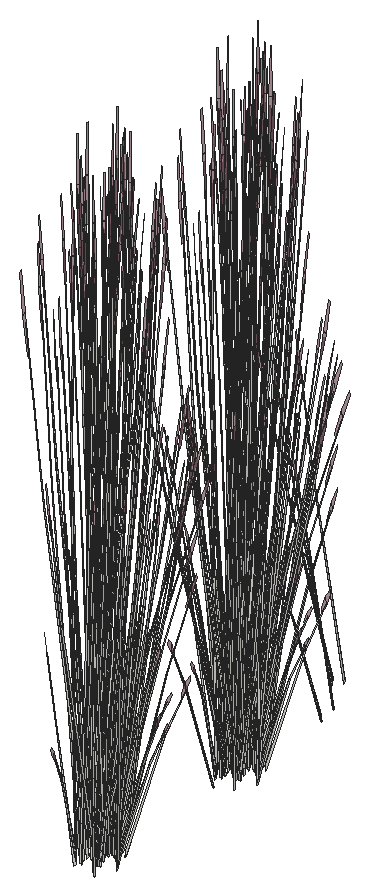
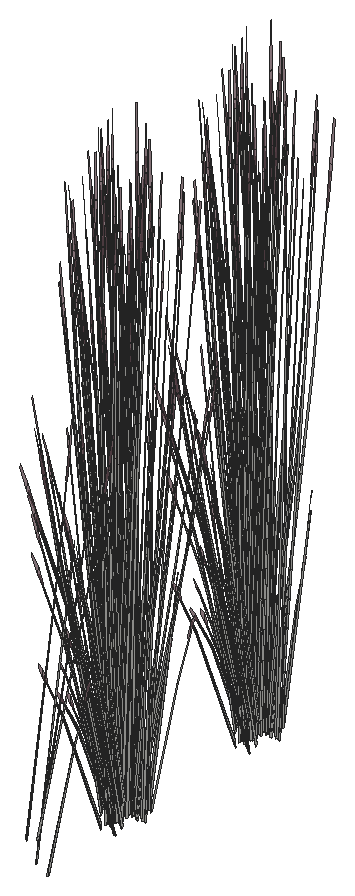
# SketchUp Ruby script. Lengths in inches.
U = 1.inch
M = Sketchup.active_model
def pt(a) = Geom::Point3d.new(a.map { |v| v * U })
def face(e, loops, mat)
  f = e.add_face(loops[0].map { |a| pt(a) })
  loops[1..].each { |l| e.add_face(l.map { |a| pt(a) }).erase! }
  f.material = f.back_material = mat if mat
  f
end
# faces: each face lists its corners as indices into pts; further lists are holes
def faces(e, pts, list, mat = nil) = list.each { |f| face(e, (f[0].is_a?(Array) ? f : [f]).map { |l| l.map { |i| pts[i] } }, mat) }
# xy, xz, yz: faces in a plane at the given z, y or x. An outline is a flat list of corners, or four numbers for a rectangle; further outlines are holes
def ring(l) = l.size == 4 ? [[l[0], l[1]], [l[2], l[1]], [l[2], l[3]], [l[0], l[3]]] : l.each_slice(2).to_a
def flat(e, list, mat, &to3) = list.each { |f| face(e, (f[0].is_a?(Array) ? f : [f]).map { |l| ring(l).map { |u, v| to3.(u, v) } }, mat) }
def xy(e, z, list, mat = nil) = flat(e, list, mat) { |x, y| [x, y, z] }
def xz(e, y, list, mat = nil) = flat(e, list, mat) { |x, z| [x, y, z] }
def yz(e, x, list, mat = nil) = flat(e, list, mat) { |y, z| [x, y, z] }
def lines(e, pts, list) = list.each { |a, b| e.add_line(pt(pts[a]), pt(pts[b])) }
# prism: a flat outline (further loops are holes) pulled along v
def prism(e, loops, v, mat = nil)
  f = face(e, loops, mat); d = Geom::Vector3d.new(v.map { |x| x * U })
  f.pushpull(f.normal.samedirection?(d) ? d.length : -d.length)
end
def box(e, o, s, mat = nil) = prism(e, [[o, [o[0] + s[0], o[1], o[2]], [o[0] + s[0], o[1] + s[1], o[2]], [o[0], o[1] + s[1], o[2]]]], [0, 0, s[2]], mat)
def at(x, y, z, deg = 0) = Geom::Transformation.translation(pt([x, y, z])) * Geom::Transformation.rotation(ORIGIN, Z_AXIS, deg.degrees)
def axes(o, x, y, z) = Geom::Transformation.new([*x, 0, *y, 0, *z, 0, *pt(o).to_a, 1])
def part(name) = M.definitions.add(name)
# library, detail: a bought-in or finely detailed component or shape, given as its bounding box
def library(name, o, s) = part(name).tap { |d| box(d.entities, o, s) }
def detail(e, o, s) = box(e.add_group.entities, o, s)
def put(e, d, t, mat = nil) = e.add_instance(d, t).tap { |i| i.material = mat if mat }
def group(e, t, mat = nil) = e.add_group.tap { |g| g.transformation = t; g.material = mat if mat }.entities
root = M.entities
M.materials.add("LightPink_Translucent").color = [144, 107, 117]
M.materials["LightPink_Translucent"].alpha = 0.75
c1 = part("blade")
p = [[2.15,0.21,22],[0,0.17,0],[0.09,0.45,0],[2.18,0.31,22],[2.29,0.31,22],[0.38,0.45,0],
  [2.48,0.24,33],[2.49,0.24,33],[2.48,0.22,33]]
faces(c1.entities,p,[[0,1,2,3],[4,5,2,3],[6,3,4,7],[8,0,3,6]])
c2 = part("seeds")
p = [[0.3,-0.1,1.38],[-0.01,-0.03,1.59],[-0.01,-0.03,0.03],[0.14,-0.07,-0.07],[0.29,-0.03,3],[0.15,0.01,3.11]]
faces(c2.entities,p,[[0,1,2,3],[1,0,4,5]],"LightPink_Translucent")
c3 = part("blade with seeds")
put(c3.entities,c1,at(0,0,0))
put(c3.entities,c2,axes([2.4,0.25,30.99],[1.5799,-0.05474,1.17369],[-0.12525,1.92788,0.29478],[-0.07173,-0.02425,1.56792]))
put(root,c3,axes([402.35,721.51,2.77],[0.04528,0.27194,1.1486],[-0.25117,-0.15062,0.84392],[0.02703,-0.13924,0.25299]))
put(root,c3,axes([402.89,722.82,4.68],[-0.25266,-0.31335,-0.51099],[0.2669,-0.27442,-0.3958],[0.03844,-0.15921,0.97773]))
put(root,c3,axes([403.13,722.7,4.53],[0.23881,-0.24554,-0.35414],[0.22606,0.28036,0.4572],[0.0344,-0.14245,0.87481]))
put(root,c3,axes([401.49,724.01,2.1],[-0.14494,-0.47823,-0.69835],[0.41752,-0.17223,-0.18329],[-0.01602,-0.16194,1.54149]))
put(root,c3,axes([403.43,722.55,1.49],[-0.05283,-0.03674,1.76342],[-0.13569,-0.41045,-0.26939],[0.09154,-0.11138,0.30037]))
put(root,c3,axes([403.42,723.71,4.98],[0.18436,-0.36797,-0.71045],[0.32306,0.26151,0.08574],[0.11008,-0.13332,1.00501]))
put(root,c3,axes([401.43,722.64,2.375],[-0.22066,-0.46731,0],[0.36918,-0.26061,-0.51607],[0.08408,-0.05936,1.63711]))
put(root,c3,axes([403.41,723.54,4.68],[-0.09067,-0.42583,-0.51099],[0.34336,-0.07449,-0.3958],[0.0984,-0.11438,0.97773]))
put(root,c3,axes([401.92,722.07,2.13],[-0.2439,0.26754,-0.03893],[-0.22348,-0.29302,-0.17649],[-0.01573,-0.08303,0.58215]))
put(root,c3,axes([400.63,723.95,2.02],[0,-0.46636,-0.49651],[0.39487,0,0],[0,-0.10622,1.57504]))
put(root,c3,axes([401.73,722.57,2.02],[0.33032,-0.23318,-0.49651],[0.19744,0.41812,0],[0.07523,-0.05311,1.57504]))
put(root,c3,axes([403.69,723.37,2.59],[-0.12609,-0.01381,1.43002],[-0.12917,-0.37055,-0.30754],[0.1549,-0.10482,0.61141]))
put(root,c3,axes([402.12,723.52,2.06],[0.23773,-0.35053,-0.62353],[0.29532,0.31785,-0.16365],[0.09526,-0.08744,1.37633]))
put(root,c3,axes([403.84,722.69,2.77],[-0.11756,0.2374,1.1486],[-0.10105,-0.31895,0.84392],[0.09709,-0.07992,0.25299]))
put(root,c3,axes([403.67,723.58,4.53],[0.30722,-0.06665,-0.35414],[0.08112,0.381,0.4572],[0.08804,-0.10234,0.87481]))
put(root,c3,axes([401.71,724.14,2.21],[0.17124,-0.42022,-0.44739],[0.35581,0.20224,0.21531],[0,-0.09687,1.43643]))
put(root,c3,axes([401.86,723.93,2.67],[-0.04113,-0.53214,-0.29095],[0.42835,-0.03218,-0.50002],[0.07543,-0.07088,1.59708]))
put(root,c3,axes([400.8,723.96,2.03],[0.24637,-0.29097,-0.30978],[0.24637,0.29097,0.30978],[0,-0.09372,1.38974]))
put(root,c3,axes([401.67,724.49,2.67],[-0.39748,-0.22252,-0.29095],[0.19139,-0.46966,-0.50002],[-0.01249,-0.11531,1.59708]))
put(root,c3,axes([401.81,722.75,2.03],[0.32928,0.11539,-0.30978],[-0.08291,0.40636,0.30978],[0.06638,-0.04686,1.38974]))
put(root,c3,axes([401.92,724.34,2.43],[0.39767,0.22603,0.24065],[-0.19139,0.46966,0.50002],[0,-0.10827,1.60543]))
put(root,c3,axes([401.79,724.03,2.72],[-0.38326,0.02879,0.44739],[-0.03466,-0.47788,-0.21531],[0.06861,-0.04843,1.43643]))
put(root,c3,axes([400.8,724.38,2.48],[0,0.46636,0.49651],[-0.39487,0,0],[0,-0.10622,1.57504]))
put(root,c3,axes([403.57,724.48,4.68],[0.09562,-0.42421,-0.51099],[0.32782,0.1454,-0.3958],[0.13199,-0.0389,0.97773]))
put(root,c3,axes([403.06,722.76,2.375],[0.22066,-0.46731,0],[0.36918,0.26061,-0.51607],[0.08408,0.05936,1.63711]))
put(root,c3,axes([401.78,724.2,2.36],[0.15345,0.52148,0.45755],[-0.43845,0.18134,0.17955],[0.00536,-0.09582,1.58856]))
put(root,c3,axes([403.92,724.6,1.98],[-0.22732,0.05597,1.41583],[-0.03618,-0.44548,0.08104],[0.15921,-0.06743,0.80566]))
put(root,c3,axes([404.34,724.21,2.26],[-0.21881,-0.29821,-0.06488],[0.23965,-0.27324,-0.29416],[0.0679,-0.01924,0.97024]))
put(root,c3,axes([401.7,724.61,2.72],[-0.17124,0.42022,0.44739],[-0.35581,-0.20224,-0.21531],[0,-0.09687,1.43643]))
put(root,c3,axes([402.33,724.25,2.21],[0,-0.53961,0],[0.44133,0,0],[0,0,1.79456]))
put(root,c3,axes([402.87,723,2.48],[-0.33032,-0.23318,0.49651],[0.19744,-0.41812,0],[0.07523,0.05311,1.57504]))
put(root,c3,axes([403.51,724.64,4.98],[0.31014,-0.20596,-0.71045],[0.17284,0.42397,0.08574],[0.14985,-0.04816,1.00501]))
put(root,c3,axes([402.12,723.91,2.36],[-0.29264,0.42323,0.45755],[-0.34767,-0.3736,0.17955],[0.07055,-0.04224,1.58856]))
put(root,c3,axes([402.44,724.66,2.3],[-0.32829,-0.4014,-0.06131],[0.32849,-0.40164,0],[-0.01146,-0.01402,1.75571]))
put(root,c3,axes([401.61,723.21,2.47],[-0.10196,0.46348,0.17642],[-0.3731,-0.13116,0.35086],[0.06445,-0.00226,1.60407]))
put(root,c3,axes([401.46,723.58,1.59],[-0.3474,0.18671,1.28929],[-0.11057,-0.53572,0.50096],[0.21332,0.00891,1.46642]))
put(root,c3,axes([402.39,723.72,2.62],[0.06809,-0.4162,0.1448],[0.33266,0.07225,-0.41347],[0.06054,0.04274,1.26744]))
put(root,c3,axes([401.82,724.71,2.36],[0.44609,0.09826,0.45755],[-0.09078,0.55493,0.17955],[-0.06519,-0.05359,1.58856]))
put(root,c3,axes([404.17,724.3125,1.49],[-0.01845,-0.0708,1.76342],[0.12793,-0.41416,-0.26939],[0.12905,-0.00596,0.30037]))
put(root,c3,axes([402.25,723.83,2.72],[-0.21202,-0.39143,0.44739],[0.32115,-0.27564,-0.21531],[0.06861,0.04843,1.43643]))
put(root,c3,axes([401.58,725.6,2.47],[0.37926,-0.12378,0.17642],[0.09365,0.46065,0.35086],[-0.03382,-0.06712,1.60407]))
put(root,c3,axes([402.36,723.86,2.67],[0.35635,-0.30962,-0.29095],[0.23697,0.43749,-0.50002],[0.08792,0.04443,1.59708]))
put(root,c3,axes([403.78,724.68,4.53],[0.29332,0.1301,-0.35414],[-0.08555,0.37955,0.4572],[0.11809,-0.0348,0.87481]))
put(root,c3,axes([403.26,723.04,2.02],[0.33032,0.23318,-0.49651],[-0.19744,0.41812,0],[0.07523,0.05311,1.57504]))
put(root,c3,axes([402.63,724.37,2.21],[0.39487,0,0],[0,0.48281,0],[0,0,1.78407]))
put(root,c3,axes([402.74,723.23,2.47],[-0.37926,0.12378,0.17642],[-0.09365,-0.46065,0.35086],[0.03382,0.06712,1.60407]))
put(root,c3,axes([402.98,724.21,3.875],[-0.14639,0.01056,1.71376],[0.09712,-0.45778,0.13857],[0.20862,0.02831,0.73262]))
put(root,c3,axes([403.17,723.21,2.03],[0.08291,0.40636,-0.30978],[-0.32928,0.11539,0.30978],[0.06638,0.04686,1.38974]))
put(root,c3,axes([402.5,724.12,2.38],[-0.44609,-0.09826,0.49198],[0.09078,-0.55493,0.19306],[0.06519,0.05359,1.70813]))
put(root,c3,axes([402.15,725.49,2.2],[-0.11516,-0.40207,0],[0.32884,-0.1408,0],[0,0,1.54371]))
put(root,c3,axes([402.58,725.43,2.18],[0.37054,-0.15823,-0.19198],[0.1302,0.45581,0.00008],[0.0409,-0.01749,1.73897]))
put(root,c3,axes([402.71,725.625,2.47],[0.10196,-0.46348,0.17642],[0.3731,0.13116,0.35086],[-0.06445,0.00226,1.60407]))
put(root,c3,axes([402.62,724.57,2.21],[0.24637,0.30123,0],[-0.24637,0.30123,0],[0,0,1.69266]))
put(root,c3,axes([403.29,724.44,2.47],[-0.2773,-0.3397,0.17642],[0.27945,-0.32949,0.35086],[-0.03063,0.06937,1.60407]))
put(root,c3,axes([402.78,723.93,2.06],[0.36714,0.07646,-0.62353],[-0.07747,0.47163,-0.16365],[0.10956,0.05715,1.37633]))
put(root,c3,axes([404.4,724.75,2.77],[-0.21807,0.07699,1.1486],[0.10265,-0.31819,0.84392],[0.11568,0.02177,0.25299]))
put(root,c3,axes([402.07,725.67,2.2],[-0.35581,-0.20937,0],[0.17124,-0.43505,0],[0,0,1.62707]))
put(root,c3,axes([402.62,724.22,2.72],[0.17124,-0.42022,0.44739],[0.35581,0.20224,-0.21531],[0,0.09687,1.43643]))
put(root,c3,axes([402.55,724.46,2.29],[0,0.53934,-0.05637],[-0.44133,0,0],[0,0.01695,1.79368]))
put(root,c3,axes([402.58,724.08,2.21],[0.21202,0.39143,-0.44739],[-0.32115,0.27564,0.21531],[0.06861,0.04843,1.43643]))
put(root,c3,axes([404.02,725.73,3.93],[-0.06755,-0.39203,-0.03492],[0.31928,-0.09013,-0.15832],[0.06667,0.02485,0.52218]))
put(root,c3,axes([403.52,724.46,2.48],[0,-0.46636,0.49651],[0.39487,0,0],[0,0.10622,1.57504]))
put(root,c3,axes([402.53,724.8,2.72],[0.38326,-0.02879,0.44739],[0.03466,0.47788,-0.21531],[-0.06861,0.04843,1.43643]))
put(root,c3,axes([402.77,724.32,2.62],[0.32884,-0.136,0.1448],[0.11516,0.38837,-0.41347],[0,0.08547,1.26744]))
put(root,c3,axes([403.99,725.26,2.59],[-0.085,-0.1147,1.43002],[0.1106,-0.37943,-0.30754],[0.17198,0.0514,0.61141]))
put(root,c3,axes([402.47,725.68,2.2],[0.35581,0.20937,0],[-0.17124,0.43505,0],[0,0,1.74954]))
put(root,c3,axes([402.61,726.14,2.19],[-0.21791,-0.46895,-0.05142],[0.36918,-0.26061,0.51607],[-0.09097,0.04465,1.6363]))
put(root,c3,axes([402.53,725.01,2.62],[0.26075,0.2802,0.1448],[-0.2175,0.31612,-0.41347],[-0.06054,0.04274,1.26744]))
put(root,c3,axes([403.21,725.49,4.98],[0.35281,0.01123,-0.71045],[-0.0237,0.47284,0.08574],[0.14947,0.0499,1.00501]))
put(root,c3,axes([402.8125,725.875,2.48],[0.33032,-0.23318,0.49651],[0.19744,0.41812,0],[-0.07523,0.05311,1.57504]))
put(root,c3,axes([402.34,725.51,2.29],[0.15345,0.53576,-0.06012],[-0.43845,0.18773,0],[0.00536,0.01871,1.72173]))
put(root,c3,axes([402.51,726.08,2.03],[-0.32928,-0.11539,-0.30978],[0.08291,-0.40636,0.30978],[-0.06638,0.04686,1.38974]))
put(root,c3,axes([403.78,724.53,2.375],[0.44133,0,0],[0,0.52122,-0.51607],[0,0.11871,1.63711]))
put(root,c3,axes([403.61,724.8,2.2],[-0.44111,-0.00373,-0.04976],[0,-0.52122,0.49943],[-0.01386,0.11865,1.58352]))
put(root,c3,axes([402.65,724.35,2.67],[0.39748,0.22252,-0.29095],[-0.19139,0.46966,-0.50002],[0.01249,0.11531,1.59708]))
put(root,c3,axes([403.42,725.6875,4.53],[0.20082,0.29199,-0.35414],[-0.2293,0.2764,0.4572],[0.1165,0.04206,0.87481]))
put(root,c3,axes([403.52,724.88,2.03],[-0.24637,0.29097,-0.30978],[-0.24637,-0.29097,0.30978],[0,0.09372,1.38974]))
put(root,c3,axes([402.46,724.91,2.67],[0.04113,0.53214,-0.29095],[-0.42835,0.03218,-0.50002],[-0.07543,0.07088,1.59708]))
put(root,c3,axes([402.61,724.7,2.21],[-0.17124,0.42022,-0.44739],[-0.35581,-0.20224,0.21531],[0,0.09687,1.43643]))
put(root,c3,axes([402.62,725.9,2.33],[0.44186,0.15158,0.30756],[-0.11054,0.54181,-0.36492],[-0.07313,0.06781,1.64885]))
put(root,c3,axes([402.59,726.27,2.02],[-0.33032,0.23318,-0.49651],[-0.19744,-0.41812,0],[-0.07523,0.05311,1.57504]))
put(root,c3,axes([403.6875,724.89,2.02],[0,0.46636,-0.49651],[-0.39487,0,0],[0,0.10622,1.57504]))
put(root,c3,axes([402.7,724.94,3.875],[-0.1311,-0.08035,1.71376],[0.27131,-0.33708,0.13857],[0.16909,0.15206,0.73262]))
put(root,c3,axes([403.18,725.86,2.77],[-0.19872,-0.13409,1.1486],[0.2566,-0.13625,0.84392],[0.06921,0.11541,0.25299]))
put(root,c3,axes([402.89,726.2,2.375],[0.22066,0.46731,0],[-0.36918,0.26061,-0.51607],[-0.08408,0.05936,1.63711]))
put(root,c3,axes([403.24,726.35,1.49],[0.02571,-0.06733,1.76342],[0.32373,-0.19829,-0.26939],[0.09815,0.10263,0.30037]))
put(root,c3,axes([402.7,724.35,2.84],[-0.00964,-0.43909,1.41272],[0.43635,0.11382,0.59816],[-0.1032,0.24027,1.3335]))
put(root,c3,axes([402.8125,724.82,2.09],[0.12941,0.42699,-0.69212],[-0.37279,0.15378,-0.18165],[0.0143,0.14459,1.52773]))
put(root,c3,axes([402.74,726.04,4.68],[0.34827,-0.11086,-0.51099],[0.06092,0.41983,-0.3958],[0.09354,0.12031,0.97773]))
put(root,c3,axes([403.22,726.47,2.67],[-0.22633,-0.01463,1.0506],[0.14947,-0.31064,0.58006],[0.08941,0.11036,0.8241]))
put(root,c3,axes([402.48,725.71,2.59],[0.00623,-0.15459,1.43002],[0.29764,-0.17268,-0.30754],[0.09188,0.18503,0.61141]))
put(root,c3,axes([401.73,726.34,1.49],[0.05712,-0.02538,1.76342],[0.34359,0.13968,-0.26939],[0.01005,0.15742,0.30037]))
put(root,c3,axes([401.21,725.93,5],[0.25266,0.31335,-0.5672],[-0.2669,0.27442,-0.43934],[-0.03844,0.15921,1.08528]))
put(root,c3,axes([400.9375,726.4,2.82],[0.32063,-0.08258,0.06507],[0.07371,0.33271,-0.86304],[-0.02033,0.16842,0.7736]))
put(root,c3,axes([401.96,726.24,4.68],[0.34695,0.11691,-0.51099],[-0.11892,0.40083,-0.3958],[0.03181,0.16138,0.97773]))
put(root,c3,axes([402.16,725.41,3.875],[-0.08068,-0.14973,1.71376],[0.3728,-0.12606,0.13857],[0.08426,0.23506,0.73262]))
put(root,c3,axes([401.8,726.48,4.53],[-0.1064,0.35863,-0.35414],[-0.31043,-0.1046,0.4572],[0.02846,0.14439,0.87481]))
put(root,c3,axes([401.5,725.48,3.875],[-0.00864,-0.17899,1.71376],[0.37441,0.11874,0.13857],[-0.02316,0.25508,0.73262]))
put(root,c3,axes([401.84,726.16,4.98],[0.16845,0.3792,-0.71045],[-0.34676,0.21133,0.08574],[0.03939,0.18322,1.00501]))
put(root,c3,axes([402.72,739.41,2.59],[-0.10032,0.0944,1.43002],[-0.30046,-0.16522,-0.30754],[0.05569,-0.20547,0.61141]))
put(root,c3,axes([402.27,739.73,4.98],[-0.16845,-0.3792,-0.71045],[0.34676,-0.21133,0.08574],[-0.03939,-0.18322,1.00501]))
put(root,c3,axes([401.98,738.89,1.49],[-0.0592,0.0168,1.76342],[-0.32738,-0.18913,-0.26939],[0.00549,-0.15776,0.30037]))
put(root,c3,axes([402.97,740.11,4.98],[0.00918,-0.43138,-0.71045],[0.38672,0.02897,0.08574],[0.04081,-0.18275,1.00501]))
put(root,c3,axes([402.3,739.41,4.53],[0.1064,-0.35863,-0.35414],[0.31043,0.1046,0.4572],[-0.02846,-0.14439,0.87481]))
put(root,c3,axes([402.53,739.89,3.875],[-0.06572,0.16029,1.71376],[-0.27569,-0.33172,0.13857],[0.12437,-0.20675,0.73262]))
put(root,c3,axes([402.14,739.66,4.68],[-0.34695,-0.11691,-0.51099],[0.11892,-0.40083,-0.3958],[-0.03181,-0.16138,0.97773]))
put(root,c3,axes([402.35,738.65,2.77],[0.04528,0.27194,1.1486],[-0.25117,-0.15062,0.84392],[0.02703,-0.13924,0.25299]))
put(root,c3,axes([402.89,739.96,4.68],[-0.25266,-0.31335,-0.51099],[0.2669,-0.27442,-0.3958],[0.03844,-0.15921,0.97773]))
put(root,c3,axes([403.13,739.85,4.53],[0.23881,-0.24554,-0.35414],[0.22606,0.28036,0.4572],[0.0344,-0.14245,0.87481]))
put(root,c3,axes([401.49,741.16,2.1],[-0.14494,-0.47823,-0.69835],[0.41752,-0.17223,-0.18329],[-0.01602,-0.16194,1.54149]))
put(root,c3,axes([403.43,739.7,1.49],[-0.05283,-0.03674,1.76342],[-0.13569,-0.41045,-0.26939],[0.09154,-0.11138,0.30037]))
put(root,c3,axes([403.42,740.86,4.98],[0.18436,-0.36797,-0.71045],[0.32306,0.26151,0.08574],[0.11008,-0.13332,1.00501]))
put(root,c3,axes([401.43,739.78,2.375],[-0.22066,-0.46731,0],[0.36918,-0.26061,-0.51607],[0.08408,-0.05936,1.63711]))
put(root,c3,axes([403.41,740.68,4.68],[-0.09067,-0.42583,-0.51099],[0.34336,-0.07449,-0.3958],[0.0984,-0.11438,0.97773]))
put(root,c3,axes([401.92,739.22,2.13],[-0.2439,0.26754,-0.03893],[-0.22348,-0.29302,-0.17649],[-0.01573,-0.08303,0.58215]))
put(root,c3,axes([400.63,741.09,2.02],[0,-0.46636,-0.49651],[0.39487,0,0],[0,-0.10622,1.57504]))
put(root,c3,axes([401.73,739.71,2.02],[0.33032,-0.23318,-0.49651],[0.19744,0.41812,0],[0.07523,-0.05311,1.57504]))
put(root,c3,axes([403.69,740.52,2.59],[-0.12609,-0.01381,1.43002],[-0.12917,-0.37055,-0.30754],[0.1549,-0.10482,0.61141]))
put(root,c3,axes([402.12,740.67,2.06],[0.23773,-0.35053,-0.62353],[0.29532,0.31785,-0.16365],[0.09526,-0.08744,1.37633]))
put(root,c3,axes([403.84,739.84,2.77],[-0.11756,0.2374,1.1486],[-0.10105,-0.31895,0.84392],[0.09709,-0.07992,0.25299]))
put(root,c3,axes([403.67,740.73,4.53],[0.30722,-0.06665,-0.35414],[0.08112,0.381,0.4572],[0.08804,-0.10234,0.87481]))
put(root,c3,axes([401.71,741.28,2.21],[0.17124,-0.42022,-0.44739],[0.35581,0.20224,0.21531],[0,-0.09687,1.43643]))
put(root,c3,axes([401.86,741.07,2.67],[-0.04113,-0.53214,-0.29095],[0.42835,-0.03218,-0.50002],[0.07543,-0.07088,1.59708]))
put(root,c3,axes([400.8,741.1,2.03],[0.24637,-0.29097,-0.30978],[0.24637,0.29097,0.30978],[0,-0.09372,1.38974]))
put(root,c3,axes([401.67,741.63,2.67],[-0.39748,-0.22252,-0.29095],[0.19139,-0.46966,-0.50002],[-0.01249,-0.11531,1.59708]))
put(root,c3,axes([401.81,739.9,2.03],[0.32928,0.11539,-0.30978],[-0.08291,0.40636,0.30978],[0.06638,-0.04686,1.38974]))
put(root,c3,axes([401.92,741.49,2.43],[0.39767,0.22603,0.24065],[-0.19139,0.46966,0.50002],[0,-0.10827,1.60543]))
put(root,c3,axes([401.79,741.18,2.72],[-0.38326,0.02879,0.44739],[-0.03466,-0.47788,-0.21531],[0.06861,-0.04843,1.43643]))
put(root,c3,axes([400.8,741.53,2.48],[0,0.46636,0.49651],[-0.39487,0,0],[0,-0.10622,1.57504]))
put(root,c3,axes([403.57,741.63,4.68],[0.09562,-0.42421,-0.51099],[0.32782,0.1454,-0.3958],[0.13199,-0.0389,0.97773]))
put(root,c3,axes([403.06,739.9,2.375],[0.22066,-0.46731,0],[0.36918,0.26061,-0.51607],[0.08408,0.05936,1.63711]))
put(root,c3,axes([401.78,741.35,2.36],[0.15345,0.52148,0.45755],[-0.43845,0.18134,0.17955],[0.00536,-0.09582,1.58856]))
put(root,c3,axes([403.92,741.75,1.98],[-0.22732,0.05597,1.41583],[-0.03618,-0.44548,0.08104],[0.15921,-0.06743,0.80566]))
put(root,c3,axes([404.34,741.35,2.26],[-0.21881,-0.29821,-0.06488],[0.23965,-0.27324,-0.29416],[0.0679,-0.01924,0.97024]))
put(root,c3,axes([401.7,741.76,2.72],[-0.17124,0.42022,0.44739],[-0.35581,-0.20224,-0.21531],[0,-0.09687,1.43643]))
put(root,c3,axes([402.33,741.39,2.21],[0,-0.53961,0],[0.44133,0,0],[0,0,1.79456]))
put(root,c3,axes([402.87,740.15,2.48],[-0.33032,-0.23318,0.49651],[0.19744,-0.41812,0],[0.07523,0.05311,1.57504]))
put(root,c3,axes([403.51,741.78,4.98],[0.31014,-0.20596,-0.71045],[0.17284,0.42397,0.08574],[0.14985,-0.04816,1.00501]))
put(root,c3,axes([402.12,741.05,2.36],[-0.29264,0.42323,0.45755],[-0.34767,-0.3736,0.17955],[0.07055,-0.04224,1.58856]))
put(root,c3,axes([402.44,741.8125,2.3],[-0.32829,-0.4014,-0.06131],[0.32849,-0.40164,0],[-0.01146,-0.01402,1.75571]))
put(root,c3,axes([401.61,740.36,2.47],[-0.10196,0.46348,0.17642],[-0.3731,-0.13116,0.35086],[0.06445,-0.00226,1.60407]))
put(root,c3,axes([401.46,740.73,1.59],[-0.3474,0.18671,1.28929],[-0.11057,-0.53572,0.50096],[0.21332,0.00891,1.46642]))
put(root,c3,axes([402.39,740.87,2.62],[0.06809,-0.4162,0.1448],[0.33266,0.07225,-0.41347],[0.06054,0.04274,1.26744]))
put(root,c3,axes([401.82,741.86,2.36],[0.44609,0.09826,0.45755],[-0.09078,0.55493,0.17955],[-0.06519,-0.05359,1.58856]))
put(root,c3,axes([404.17,741.46,1.49],[-0.01845,-0.0708,1.76342],[0.12793,-0.41416,-0.26939],[0.12905,-0.00596,0.30037]))
put(root,c3,axes([402.25,740.98,2.72],[-0.21202,-0.39143,0.44739],[0.32115,-0.27564,-0.21531],[0.06861,0.04843,1.43643]))
put(root,c3,axes([401.58,742.75,2.47],[0.37926,-0.12378,0.17642],[0.09365,0.46065,0.35086],[-0.03382,-0.06712,1.60407]))
put(root,c3,axes([402.36,741.01,2.67],[0.35635,-0.30962,-0.29095],[0.23697,0.43749,-0.50002],[0.08792,0.04443,1.59708]))
put(root,c3,axes([403.78,741.82,4.53],[0.29332,0.1301,-0.35414],[-0.08555,0.37955,0.4572],[0.11809,-0.0348,0.87481]))
put(root,c3,axes([403.26,740.18,2.02],[0.33032,0.23318,-0.49651],[-0.19744,0.41812,0],[0.07523,0.05311,1.57504]))
put(root,c3,axes([402.63,741.51,2.21],[0.39487,0,0],[0,0.48281,0],[0,0,1.78407]))
put(root,c3,axes([402.74,740.38,2.47],[-0.37926,0.12378,0.17642],[-0.09365,-0.46065,0.35086],[0.03382,0.06712,1.60407]))
put(root,c3,axes([402.98,741.35,3.875],[-0.14639,0.01056,1.71376],[0.09712,-0.45778,0.13857],[0.20862,0.02831,0.73262]))
put(root,c3,axes([403.17,740.36,2.03],[0.08291,0.40636,-0.30978],[-0.32928,0.11539,0.30978],[0.06638,0.04686,1.38974]))
put(root,c3,axes([402.5,741.27,2.38],[-0.44609,-0.09826,0.49198],[0.09078,-0.55493,0.19306],[0.06519,0.05359,1.70813]))
put(root,c3,axes([402.15,742.64,2.2],[-0.11516,-0.40207,0],[0.32884,-0.1408,0],[0,0,1.54371]))
put(root,c3,axes([402.58,742.58,2.18],[0.37054,-0.15823,-0.19198],[0.1302,0.45581,0.00008],[0.0409,-0.01749,1.73897]))
put(root,c3,axes([402.71,742.77,2.47],[0.10196,-0.46348,0.17642],[0.3731,0.13116,0.35086],[-0.06445,0.00226,1.60407]))
put(root,c3,axes([402.62,741.72,2.21],[0.24637,0.30123,0],[-0.24637,0.30123,0],[0,0,1.69266]))
put(root,c3,axes([403.29,741.59,2.47],[-0.2773,-0.3397,0.17642],[0.27945,-0.32949,0.35086],[-0.03063,0.06937,1.60407]))
put(root,c3,axes([402.78,741.08,2.06],[0.36714,0.07646,-0.62353],[-0.07747,0.47163,-0.16365],[0.10956,0.05715,1.37633]))
put(root,c3,axes([404.4,741.9,2.77],[-0.21807,0.07699,1.1486],[0.10265,-0.31819,0.84392],[0.11568,0.02177,0.25299]))
put(root,c3,axes([402.07,742.82,2.2],[-0.35581,-0.20937,0],[0.17124,-0.43505,0],[0,0,1.62707]))
put(root,c3,axes([402.62,741.37,2.72],[0.17124,-0.42022,0.44739],[0.35581,0.20224,-0.21531],[0,0.09687,1.43643]))
put(root,c3,axes([402.55,741.61,2.29],[0,0.53934,-0.05637],[-0.44133,0,0],[0,0.01695,1.79368]))
put(root,c3,axes([402.58,741.23,2.21],[0.21202,0.39143,-0.44739],[-0.32115,0.27564,0.21531],[0.06861,0.04843,1.43643]))
put(root,c3,axes([404.02,742.88,3.93],[-0.06755,-0.39203,-0.03492],[0.31928,-0.09013,-0.15832],[0.06667,0.02485,0.52218]))
put(root,c3,axes([403.52,741.6,2.48],[0,-0.46636,0.49651],[0.39487,0,0],[0,0.10622,1.57504]))
put(root,c3,axes([402.53,741.95,2.72],[0.38326,-0.02879,0.44739],[0.03466,0.47788,-0.21531],[-0.06861,0.04843,1.43643]))
put(root,c3,axes([402.77,741.46,2.62],[0.32884,-0.136,0.1448],[0.11516,0.38837,-0.41347],[0,0.08547,1.26744]))
put(root,c3,axes([403.99,742.41,2.59],[-0.085,-0.1147,1.43002],[0.1106,-0.37943,-0.30754],[0.17198,0.0514,0.61141]))
put(root,c3,axes([402.47,742.83,2.2],[0.35581,0.20937,0],[-0.17124,0.43505,0],[0,0,1.74954]))
put(root,c3,axes([402.61,743.29,2.19],[-0.21791,-0.46895,-0.05142],[0.36918,-0.26061,0.51607],[-0.09097,0.04465,1.6363]))
put(root,c3,axes([402.53,742.16,2.62],[0.26075,0.2802,0.1448],[-0.2175,0.31612,-0.41347],[-0.06054,0.04274,1.26744]))
put(root,c3,axes([403.21,742.64,4.98],[0.35281,0.01123,-0.71045],[-0.0237,0.47284,0.08574],[0.14947,0.0499,1.00501]))
put(root,c3,axes([402.8125,743.02,2.48],[0.33032,-0.23318,0.49651],[0.19744,0.41812,0],[-0.07523,0.05311,1.57504]))
put(root,c3,axes([402.34,742.65,2.29],[0.15345,0.53576,-0.06012],[-0.43845,0.18773,0],[0.00536,0.01871,1.72173]))
put(root,c3,axes([402.51,743.23,2.03],[-0.32928,-0.11539,-0.30978],[0.08291,-0.40636,0.30978],[-0.06638,0.04686,1.38974]))
put(root,c3,axes([403.78,741.68,2.375],[0.44133,0,0],[0,0.52122,-0.51607],[0,0.11871,1.63711]))
put(root,c3,axes([403.61,741.95,2.2],[-0.44111,-0.00373,-0.04976],[0,-0.52122,0.49943],[-0.01386,0.11865,1.58352]))
put(root,c3,axes([402.65,741.5,2.67],[0.39748,0.22252,-0.29095],[-0.19139,0.46966,-0.50002],[0.01249,0.11531,1.59708]))
put(root,c3,axes([403.42,742.84,4.53],[0.20082,0.29199,-0.35414],[-0.2293,0.2764,0.4572],[0.1165,0.04206,0.87481]))
put(root,c3,axes([403.52,742.02,2.03],[-0.24637,0.29097,-0.30978],[-0.24637,-0.29097,0.30978],[0,0.09372,1.38974]))
put(root,c3,axes([402.46,742.05,2.67],[0.04113,0.53214,-0.29095],[-0.42835,0.03218,-0.50002],[-0.07543,0.07088,1.59708]))
put(root,c3,axes([402.61,741.84,2.21],[-0.17124,0.42022,-0.44739],[-0.35581,-0.20224,0.21531],[0,0.09687,1.43643]))
put(root,c3,axes([402.62,743.05,2.33],[0.44186,0.15158,0.30756],[-0.11054,0.54181,-0.36492],[-0.07313,0.06781,1.64885]))
put(root,c3,axes([402.59,743.42,2.02],[-0.33032,0.23318,-0.49651],[-0.19744,-0.41812,0],[-0.07523,0.05311,1.57504]))
put(root,c3,axes([403.6875,742.04,2.02],[0,0.46636,-0.49651],[-0.39487,0,0],[0,0.10622,1.57504]))
put(root,c3,axes([402.7,742.09,3.875],[-0.1311,-0.08035,1.71376],[0.27131,-0.33708,0.13857],[0.16909,0.15206,0.73262]))
put(root,c3,axes([403.18,743,2.77],[-0.19872,-0.13409,1.1486],[0.2566,-0.13625,0.84392],[0.06921,0.11541,0.25299]))
put(root,c3,axes([402.89,743.34,2.375],[0.22066,0.46731,0],[-0.36918,0.26061,-0.51607],[-0.08408,0.05936,1.63711]))
put(root,c3,axes([403.24,743.5,1.49],[0.02571,-0.06733,1.76342],[0.32373,-0.19829,-0.26939],[0.09815,0.10263,0.30037]))
put(root,c3,axes([402.7,741.49,2.84],[-0.00964,-0.43909,1.41272],[0.43635,0.11382,0.59816],[-0.1032,0.24027,1.3335]))
put(root,c3,axes([402.8125,741.97,2.09],[0.12941,0.42699,-0.69212],[-0.37279,0.15378,-0.18165],[0.0143,0.14459,1.52773]))
put(root,c3,axes([402.74,743.1875,4.68],[0.34827,-0.11086,-0.51099],[0.06092,0.41983,-0.3958],[0.09354,0.12031,0.97773]))
put(root,c3,axes([403.22,743.61,2.67],[-0.22633,-0.01463,1.0506],[0.14947,-0.31064,0.58006],[0.08941,0.11036,0.8241]))
put(root,c3,axes([402.48,742.86,2.59],[0.00623,-0.15459,1.43002],[0.29764,-0.17268,-0.30754],[0.09188,0.18503,0.61141]))
put(root,c3,axes([401.73,743.49,1.49],[0.05712,-0.02538,1.76342],[0.34359,0.13968,-0.26939],[0.01005,0.15742,0.30037]))
put(root,c3,axes([401.21,743.08,5],[0.25266,0.31335,-0.5672],[-0.2669,0.27442,-0.43934],[-0.03844,0.15921,1.08528]))
put(root,c3,axes([400.9375,743.55,2.82],[0.32063,-0.08258,0.06507],[0.07371,0.33271,-0.86304],[-0.02033,0.16842,0.7736]))
put(root,c3,axes([401.96,743.38,4.68],[0.34695,0.11691,-0.51099],[-0.11892,0.40083,-0.3958],[0.03181,0.16138,0.97773]))
put(root,c3,axes([402.16,742.55,3.875],[-0.08068,-0.14973,1.71376],[0.3728,-0.12606,0.13857],[0.08426,0.23506,0.73262]))
put(root,c3,axes([401.8,743.63,4.53],[-0.1064,0.35863,-0.35414],[-0.31043,-0.1046,0.4572],[0.02846,0.14439,0.87481]))
put(root,c3,axes([401.5,742.63,3.875],[-0.00864,-0.17899,1.71376],[0.37441,0.11874,0.13857],[-0.02316,0.25508,0.73262]))
put(root,c3,axes([401.84,743.31,4.98],[0.16845,0.3792,-0.71045],[-0.34676,0.21133,0.08574],[0.03939,0.18322,1.00501]))
put(root,c3,axes([402.72,752.64,2.59],[-0.10032,0.0944,1.43002],[-0.30046,-0.16522,-0.30754],[0.05569,-0.20547,0.61141]))
put(root,c3,axes([402.27,752.96,4.98],[-0.16845,-0.3792,-0.71045],[0.34676,-0.21133,0.08574],[-0.03939,-0.18322,1.00501]))
put(root,c3,axes([401.98,752.125,1.49],[-0.0592,0.0168,1.76342],[-0.32738,-0.18913,-0.26939],[0.00549,-0.15776,0.30037]))
put(root,c3,axes([402.97,753.34,4.98],[0.00918,-0.43138,-0.71045],[0.38672,0.02897,0.08574],[0.04081,-0.18275,1.00501]))
put(root,c3,axes([402.3,752.64,4.53],[0.1064,-0.35863,-0.35414],[0.31043,0.1046,0.4572],[-0.02846,-0.14439,0.87481]))
